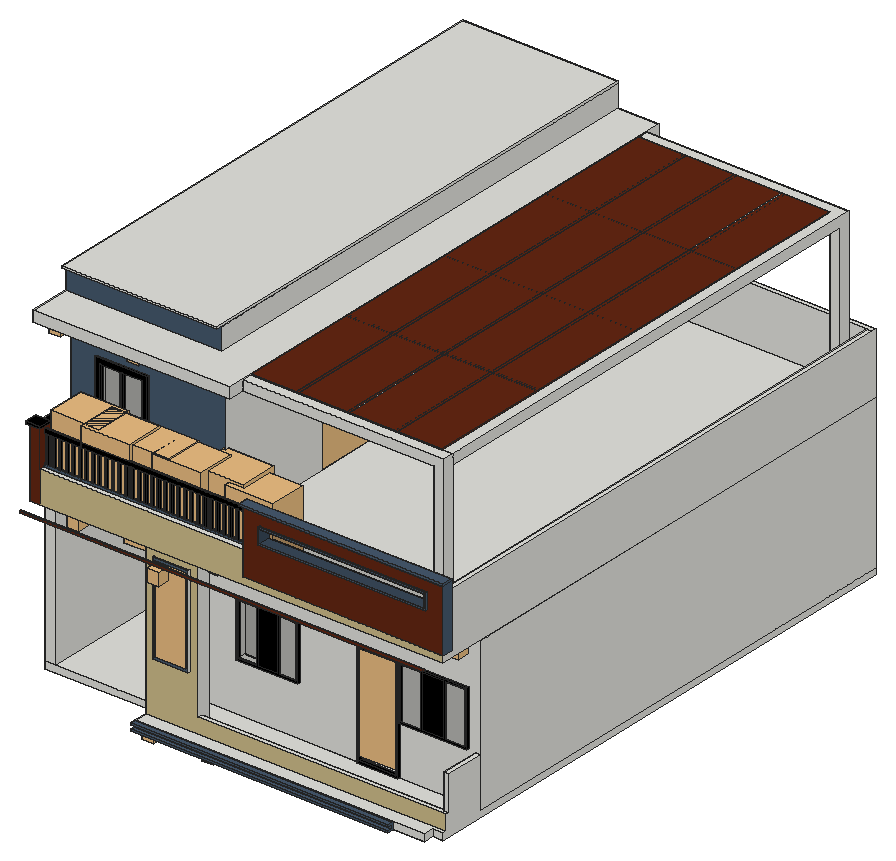
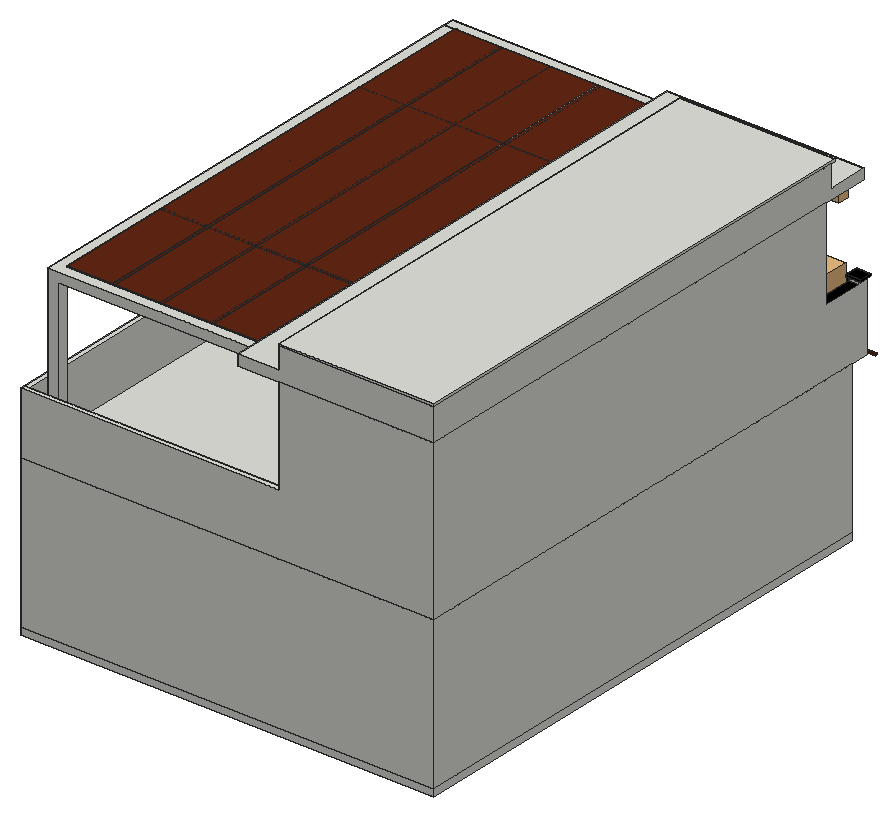
# SketchUp Ruby script. Lengths in inches.
U = 1.inch
M = Sketchup.active_model
def pt(a) = Geom::Point3d.new(a.map { |v| v * U })
def face(e, loops, mat)
  f = e.add_face(loops[0].map { |a| pt(a) })
  loops[1..].each { |l| e.add_face(l.map { |a| pt(a) }).erase! }
  f.material = f.back_material = mat if mat
  f
end
# faces: each face lists its corners as indices into pts; further lists are holes
def faces(e, pts, list, mat = nil) = list.each { |f| face(e, (f[0].is_a?(Array) ? f : [f]).map { |l| l.map { |i| pts[i] } }, mat) }
# xy, xz, yz: faces in a plane at the given z, y or x. An outline is a flat list of corners, or four numbers for a rectangle; further outlines are holes
def ring(l) = l.size == 4 ? [[l[0], l[1]], [l[2], l[1]], [l[2], l[3]], [l[0], l[3]]] : l.each_slice(2).to_a
def flat(e, list, mat, &to3) = list.each { |f| face(e, (f[0].is_a?(Array) ? f : [f]).map { |l| ring(l).map { |u, v| to3.(u, v) } }, mat) }
def xy(e, z, list, mat = nil) = flat(e, list, mat) { |x, y| [x, y, z] }
def xz(e, y, list, mat = nil) = flat(e, list, mat) { |x, z| [x, y, z] }
def yz(e, x, list, mat = nil) = flat(e, list, mat) { |y, z| [x, y, z] }
def lines(e, pts, list) = list.each { |a, b| e.add_line(pt(pts[a]), pt(pts[b])) }
# prism: a flat outline (further loops are holes) pulled along v
def prism(e, loops, v, mat = nil)
  f = face(e, loops, mat); d = Geom::Vector3d.new(v.map { |x| x * U })
  f.pushpull(f.normal.samedirection?(d) ? d.length : -d.length)
end
def box(e, o, s, mat = nil) = prism(e, [[o, [o[0] + s[0], o[1], o[2]], [o[0] + s[0], o[1] + s[1], o[2]], [o[0], o[1] + s[1], o[2]]]], [0, 0, s[2]], mat)
def at(x, y, z, deg = 0) = Geom::Transformation.translation(pt([x, y, z])) * Geom::Transformation.rotation(ORIGIN, Z_AXIS, deg.degrees)
def axes(o, x, y, z) = Geom::Transformation.new([*x, 0, *y, 0, *z, 0, *pt(o).to_a, 1])
def part(name) = M.definitions.add(name)
# library, detail: a bought-in or finely detailed component or shape, given as its bounding box
def library(name, o, s) = part(name).tap { |d| box(d.entities, o, s) }
def detail(e, o, s) = box(e.add_group.entities, o, s)
def put(e, d, t, mat = nil) = e.add_instance(d, t).tap { |i| i.material = mat if mat }
def group(e, t, mat = nil) = e.add_group.tap { |g| g.transformation = t; g.material = mat if mat }.entities
root = M.entities
M.materials.add("GLass").color = [0, 0, 0]
M.materials["GLass"].alpha = 0.1
M.materials.add("Wall Paint Fine Grain 01 Yellow 100cm").color = [207, 190, 139]
M.materials.add("Wall Paint Simple Reflective").color = [70, 89, 109]
M.materials.add("Wood Dark 02 100cm").color = [99, 39, 19]
M.materials.add("metal").color = [0, 0, 0]
c1 = library("Spot Light\#15",[-5.1,-5.1,-11.05],[10.2,10.2,11.05])
c2 = library("Spot Light\#16",[-5.1,-5.1,-11.05],[10.2,10.2,11.05])
c3 = library("Spot Light\#17",[-5.1,-5.1,-11.05],[10.2,10.2,11.05])
c4 = library("Spot Light\#18",[-5.1,-5.1,-11.05],[10.2,10.2,11.05])
c5 = library("Spot Light\#19",[-5.1,-5.1,-11.05],[10.2,10.2,11.05])
c6 = library("Door 01",[-21.26,-2.6,0],[42.52,9.29,84.25])
c7 = library("Group\#119",[0,0,0],[48,96,0.5])
c8 = library("Omni Light\#1",[-12,-12,-12],[24,24,24])
c9 = library("Spot Light\#14",[-5.1,-5.1,-11.05],[10.2,10.2,11.05])
c10 = library("Spot Light\#8",[-5.1,-5.1,-11.05],[10.2,10.2,11.05])
c11 = library("Spot Light\#9",[-5.1,-5.1,-11.05],[10.2,10.2,11.05])
c12 = library("Spot Light\#10",[-5.1,-5.1,-11.05],[10.2,10.2,11.05])
c13 = library("Spot Light\#11",[-5.1,-5.1,-11.05],[10.2,10.2,11.05])
c14 = library("Spot Light\#12",[-5.1,-5.1,-11.05],[10.2,10.2,11.05])
c15 = library("Spot Light\#13",[-5.1,-5.1,-11.05],[10.2,10.2,11.05])
c16 = part("Group\#55")
box(c16.entities,[0,0,-24],[2,1.04,24])
c17 = part("Group\#79")
box(c17.entities,[0,0,-0.2],[41.7,1.97,0.2])
c18 = part("Group\#74")
box(c18.entities,[0,0,-0.2],[39.14,1.97,0.2])
c19 = part("Group\#82")
box(c19.entities,[0,0,-0.2],[39.14,1.97,0.2])
c20 = part("Group\#76")
box(c20.entities,[0,0,-0.2],[1.8,103.4375,0.2])
c21 = part("Group\#81")
box(c21.entities,[0,0,-0.2],[1.8,104.8125,0.2])
c22 = part("Group\#78")
box(c22.entities,[0,0,-0.2],[41.7,1.97,0.2])
c23 = part("Group\#80")
box(c23.entities,[0,0,-0.2],[39.14,1.97,0.2])
c24 = part("Group\#83")
box(c24.entities,[0,0,-0.2],[1.8,101.4375,0.2])
c25 = part("Group\#73")
box(c25.entities,[0,0,0],[2.41,421.5,9])
c26 = library("Monstera deliciosa borsigiana 004",[-20.61,-16.32,0.13],[42.24,32.96,48.74])
c27 = library("Spot Light",[-5.1,-5.1,-11.05],[10.2,10.2,11.05])
c28 = library("Spot Light\#1",[-5.1,-5.1,-11.05],[10.2,10.2,11.05])
c29 = library("Spot Light\#2",[-5.1,-5.1,-11.05],[10.2,10.2,11.05])
c30 = library("Spot Light\#3",[-5.1,-5.1,-11.05],[10.2,10.2,11.05])
c31 = library("Spot Light\#4",[-5.1,-5.1,-11.05],[10.2,10.2,11.05])
c32 = library("Spot Light\#5",[-5.1,-5.1,-11.05],[10.2,10.2,11.05])
c33 = library("Spot Light\#6",[-5.1,-5.1,-11.05],[10.2,10.2,11.05])
c34 = library("Spot Light\#7",[-5.1,-5.1,-11.05],[10.2,10.2,11.05])
put(root,c1,at(303.03,225.95,293.99))
put(root,c2,at(353.32,228.8,293.99))
put(root,c3,at(414.5,235.73,293.99))
put(root,c4,at(475.25,244.97,293.99))
put(root,c5,at(536.13,248.13,293.99))
g1 = group(root,at(314.75,214.125,293.89),"Wall Paint Simple Reflective")
xy(g1,0,[[206.98,-5.03,-17.96,-3.91,-17.93,1.09,207,-0.03]],"Wall Paint Simple Reflective")
xy(g1,6.11,[[206.98,-5.03,207,-0.03,-17.93,1.09,-17.96,-3.91]],"Wall Paint Simple Reflective")
p = [[206.98,-5.03,1.35],[-17.96,-3.91,1.36],[-17.96,-3.91,0],[206.98,-5.03,0],[207,-0.03,0],[207,-0.03,6.11],
  [206.98,-5.03,6.11],[206.98,-5.03,4.77],[207,-1.03,4.77],[207,-1.03,1.35],[-17.9375,0.09,1.36],[-17.9375,0.09,4.79],
  [-17.96,-3.91,4.79],[-17.96,-3.91,6.11],[-17.93,1.09,6.11],[-17.93,1.09,0]]
faces(g1,p,[[0,1,2,3],[4,5,6,7,8,9,0,3],[2,1,10,11,12,13,14,15],[14,5,4,15],[1,0,9,10],[10,9,8,11],[13,12,7,6],[7,12,11,8]],"Wall Paint Simple Reflective")
g2 = group(root,at(197.75,215.125,294))
xy(g2,0,[[99.07,0,99.07,25.84,0,25.84,0,480,360,480,360,9,351,9,351,0]],"Wood Dark 02 100cm")
xy(g2,6,[[99.07,0,351,0,351,9,360,9,360,12,99.07,12],[144.07,16.5,355.5,16.5,355.5,49.79,360,49.79,360,480,0,480,0,25.84,99.07,25.84,99.07,23.84,144.07,23.84]])
xy(g2,19,[[144.07,12,360,12,360,14.84,355.5,14.84,355.5,16.5,144.07,16.5]])
xy(g2,49,[[355.5,14.84,360,49.79]])
xy(g2,52,[[106.07,10,137.07,12]])
xy(g2,54,[[108.07,10,135.07,23.84]])
xy(g2,129,[[108.07,10,135.07,23.84]])
xy(g2,131,[[106.07,10,137.07,12]])
xy(g2,138,[[99.07,12,144.07,23.84]])
xz(g2,0,[[99.07,0,351,6]])
xz(g2,9,[[351,0,360,6]])
xz(g2,10,[[[106.07,52,137.07,131],[108.07,54,135.07,129]]],"Wall Paint Simple Reflective")
xz(g2,12,[[[99.07,6,360,6,360,19,144.07,19,144.07,138,99.07,138],[106.07,52,137.07,131]]],"Wall Paint Fine Grain 01 Yellow 100cm")
xz(g2,14.84,[[355.5,19,360,49]])
xz(g2,16.5,[[144.07,6,355.5,19]])
xz(g2,23.84,[[[99.07,6,144.07,138],[108.07,54,135.07,129]]])
xz(g2,25.84,[[0,0,99.07,6]])
xz(g2,49.79,[[355.5,6,360,49]])
xz(g2,480,[[0,0,360,6]])
yz(g2,0,[[25.84,0,480,6]])
yz(g2,99.07,[[0,0,0,6,12,6,12,138,23.84,138,23.84,6,25.84,6,25.84,0]])
yz(g2,106.07,[[10,52,12,131]])
yz(g2,108.07,[[10,54,23.84,129]])
yz(g2,135.07,[[10,54,23.84,129]])
yz(g2,137.07,[[10,52,12,131]])
yz(g2,144.07,[[16.5,6,23.84,6,23.84,138,12,138,12,19,16.5,19]])
yz(g2,351,[[0,0,9,6]])
yz(g2,355.5,[[16.5,6,16.5,19,14.84,19,14.84,49,49.79,49,49.79,6]])
yz(g2,360,[[9,0,480,0,480,6,49.79,6,49.79,49,14.84,49,14.84,19,12,19,12,6,9,6]])
g3 = group(root,at(196.75,262.23,300))
g4 = group(g3,at(149.5,2.6875,43.44))
xy(g4,0,[[0,-1.79,54.06,0]],"metal")
xy(g4,48.89,[[0,-1.79,54.06,0]],"metal")
xz(g4,-1.79,[[[0,0,54.06,48.89],[1.8,1.63,18.02,47.26],[37.86,1.63,52.26,47.26]]],"metal")
xz(g4,0,[[[0,0,54.06,48.89],[1.8,1.63,52.26,47.26]]],"metal")
yz(g4,0,[[-1.79,0,0,48.89]],"metal")
yz(g4,1.8,[[-1.79,1.63,0,47.26]],"metal")
yz(g4,52.26,[[-1.79,1.63,0,47.26]],"metal")
yz(g4,54.06,[[-1.79,0,0,48.89]],"metal")
g5 = group(g4,at(1.8,-1.79,1.63))
box(g5,[0,0,0],[16.22,0.64,45.63],"GLass")
g6 = group(g4,at(19.82,-1.79,1.63))
box(g6,[0,0,0],[16.22,0.64,45.63],"GLass")
g7 = group(g4,at(37.86,-1.79,1.63))
box(g7,[0,0,0],[14.4,0.64,45.63],"GLass")
g8 = group(g3,at(1,2.6875,0))
xy(g8,0,[[0,-23.95,0,430.21,360,430.21,360,0,289.3,0,289.3,8.07,351,8.07,351,119.92,335.34,119.92,335.34,123.15,351,123.15,351,186.6,226.5,186.6,226.5,279.73,231,279.73,231,189.83,351,189.83,351,315.66,343.72,315.66,343.72,318.89,351,318.89,351,367.29,277.1875,367.29,277.1875,318.89,313.72,318.89,313.72,315.66,226.5,315.66,226.5,318.89,272.6875,318.89,272.6875,383.15,277.1875,383.15,277.1875,370.52,351,370.52,351,422.14,277.1875,422.14,277.1875,414.34,272.6875,414.34,272.6875,422.14,128.6875,422.14,128.6875,318.89,195,318.89,195,315.66,128.6875,315.66,128.6875,239.24,119.6875,239.24,119.6875,422.14,9,422.14,9,-23.95],[117,0,117,8.07,119.6875,8.07,119.6875,143.16,128.6875,143.16,128.6875,97.33,178.5,97.33,178.5,94.11,128.6875,94.11,128.6875,8.07,226.5,8.07,226.5,123.15,299.34,123.15,299.34,119.92,231,119.92,231,8.07,253.3,8.07,253.3,0],[119.6875,186.18,128.6875,239.24]])
xy(g8,43.44,[[148.5,0,202.5,8.07],[289.3,0,349.3,8.07]])
xy(g8,92.33,[[148.5,0,202.5,8.07],[253.3,0,349.3,8.07]])
xy(g8,96,[[178.5,94.11,226.5,97.33],[119.6875,143.16,128.6875,186.18],[226.5,279.73,231,315.66],[195,315.66,226.5,318.89],[313.72,315.66,343.72,318.89],
  [272.6875,383.15,277.1875,414.34]])
xy(g8,97.98,[[299.34,119.92,335.34,123.15]])
xy(g8,132,[[[0,-23.95,9,-23.95,9,422.14,119.6875,422.14,119.6875,8.07,117,8.07,117,0,360,0,360,430.21,0,430.21],[128.6875,97.33,128.6875,315.66,226.5,315.66,226.5,186.6,351,186.6,351,123.15,226.5,123.15,226.5,97.33],[231,189.83,351,315.66],[128.6875,318.89,272.6875,422.14],[231,8.07,351,119.92],[128.6875,8.07,226.5,94.11],[277.1875,370.52,351,422.14],[277.1875,318.89,351,367.29]]])
xz(g8,-23.95,[[0,0,9,132]])
xz(g8,0,[[[117,0,253.3,0,253.3,92.33,349.3,92.33,349.3,43.44,289.3,43.44,289.3,0,360,0,360,132,117,132],[148.5,43.44,202.5,92.33]],[172.5,43.44,202.5,92.33],[289.3,43.44,349.3,92.33]])
xz(g8,8.07,[[117,0,119.6875,132],[[128.6875,0,226.5,132],[148.5,43.44,202.5,92.33]],[231,0,231,132,351,132,351,0,289.3,0,289.3,43.44,349.3,43.44,349.3,92.33,253.3,92.33,253.3,0]])
xz(g8,94.11,[[128.6875,0,178.5,0,178.5,96,226.5,96,226.5,132,128.6875,132]])
xz(g8,97.33,[[128.6875,0,128.6875,132,226.5,132,226.5,96,178.5,96,178.5,0]])
xz(g8,119.92,[[231,0,299.34,0,299.34,97.98,335.34,97.98,335.34,0,351,0,351,132,231,132]])
xz(g8,123.15,[[226.5,0,226.5,132,351,132,351,0,335.34,0,335.34,97.98,299.34,97.98,299.34,0]])
xz(g8,143.16,[[119.6875,0,128.6875,96]])
xz(g8,186.18,[[119.6875,0,128.6875,96]])
xz(g8,186.6,[[226.5,0,351,132]])
xz(g8,189.83,[[231,0,351,132]])
xz(g8,279.73,[[226.5,0,231,96]])
xz(g8,315.66,[[128.6875,0,195,0,195,96,226.5,96,226.5,132,128.6875,132],[226.5,0,313.72,0,313.72,96,343.72,96,343.72,0,351,0,351,132,231,132,231,96,226.5,96]])
xz(g8,318.89,[[128.6875,0,128.6875,132,272.6875,132,272.6875,0,226.5,0,226.5,96,195,96,195,0],[277.1875,0,277.1875,132,351,132,351,0,343.72,0,343.72,96,313.72,96,313.72,0]])
xz(g8,367.29,[[277.1875,0,351,132]])
xz(g8,370.52,[[277.1875,0,351,132]])
xz(g8,383.15,[[272.6875,0,277.1875,96]])
xz(g8,414.34,[[272.6875,0,277.1875,96]])
xz(g8,422.14,[[9,0,119.6875,132],[128.6875,0,272.6875,132],[277.1875,0,351,132]])
xz(g8,430.21,[[0,0,360,132]])
yz(g8,0,[[-23.95,0,430.21,132]])
yz(g8,9,[[-23.95,0,422.14,132]])
yz(g8,117,[[0,0,8.07,132]])
yz(g8,119.6875,[[8.07,0,8.07,132,422.14,132,422.14,0,186.18,0,186.18,96,143.16,96,143.16,0]])
yz(g8,128.6875,[[8.07,0,94.11,132],[97.33,0,143.16,0,143.16,96,186.18,96,186.18,0,315.66,0,315.66,132,97.33,132],[318.89,0,422.14,132]])
yz(g8,178.5,[[94.11,0,97.33,96]])
yz(g8,195,[[315.66,0,318.89,96]])
yz(g8,202.5,[[0,43.44,8.07,92.33]])
yz(g8,226.5,[[8.07,0,8.07,132,94.11,132,94.11,96,97.33,96,97.33,132,123.15,132,123.15,0],[186.6,0,186.6,132,315.66,132,315.66,96,279.73,96,279.73,0],[315.66,0,318.89,96]])
yz(g8,231,[[8.07,0,119.92,132],[189.83,0,279.73,0,279.73,96,315.66,96,315.66,132,189.83,132]])
yz(g8,253.3,[[0,0,8.07,92.33]])
yz(g8,272.6875,[[318.89,0,318.89,132,422.14,132,422.14,0,414.34,0,414.34,96,383.15,96,383.15,0]])
yz(g8,277.1875,[[318.89,0,367.29,132],[370.52,0,383.15,0,383.15,96,414.34,96,414.34,0,422.14,0,422.14,132,370.52,132]])
yz(g8,289.3,[[0,0,8.07,43.44]])
yz(g8,299.34,[[119.92,0,123.15,97.98]])
yz(g8,313.72,[[315.66,0,318.89,96]])
yz(g8,335.34,[[119.92,0,123.15,97.98]])
yz(g8,343.72,[[315.66,0,318.89,96]])
yz(g8,349.3,[[0,43.44,8.07,92.33]])
yz(g8,351,[[8.07,0,119.92,132],[123.15,0,186.6,132],[189.83,0,315.66,132],[318.89,0,367.29,132],[370.52,0,422.14,132]])
yz(g8,360,[[0,0,430.21,132]])
p = [[313.72,315.66,0],[343.72,315.66,0],[226.5,279.73,0],[226.5,315.66,0],[272.6875,414.34,0],[272.6875,383.15,0],
  [195,315.66,0],[119.6875,186.18,0],[119.6875,143.16,0],[335.34,123.15,0],[299.34,123.15,0]]
lines(g8,p,[[0,1],[2,3],[4,5],[3,6],[7,8],[9,10]])
g9 = group(g8,at(253.3,0,0))
prism(g9,[[[0,1.79,0],[0,1.79,92.33],[36,1.79,92.33],[36,1.79,0]],[[34,1.79,2],[34,1.79,90.33],[2,1.79,90.33],[2,1.79,2]]],[0,-3.59,0],"metal")
g10 = group(g8,at(313.72,315.66,0))
prism(g10,[[[30,0,0],[30,0,96],[0,0,96],[0,0,0]],[[28,0,2],[2,0,2],[2,0,94],[28,0,94]]],[0,2,0])
g11 = group(g8,at(226.5,279.73,0))
prism(g11,[[[0,35.9375,0],[0,0,0],[0,0,96],[0,35.9375,96]],[[0,33.9375,94],[0,2,94],[0,2,2],[0,33.9375,2]]],[2,0,0])
g12 = group(g8,at(272.6875,383.15,0))
prism(g12,[[[0,0,0],[0,0,96],[0,31.2,96],[0,31.2,0]],[[0,2,94],[0,2,2],[0,29.2,2],[0,29.2,94]]],[2,0,0])
g13 = group(g8,at(195,315.66,0))
prism(g13,[[[0,0,96],[0,0,0],[31.5,0,0],[31.5,0,96]],[[2,0,2],[2,0,94],[29.5,0,94],[29.5,0,2]]],[0,2,0])
g14 = group(g8,at(119.6875,143.16,0))
prism(g14,[[[0,0,0],[0,0,96],[0,43.02,96],[0,43.02,0]],[[0,2,94],[0,2,2],[0,41.02,2],[0,41.02,94]]],[2,0,0])
g15 = group(g8,at(299.34,123.15,0))
prism(g15,[[[0,0,0],[0,0,97.98],[36,0,97.98],[36,0,0]],[[2,0,95.98],[2,0,2],[34,0,2],[34,0,95.98]]],[0,-2,0])
g16 = group(g3,at(290.3,2.6875,43.44))
xy(g16,0,[[0,-1.79,60,1.79]],"metal")
xy(g16,48.89,[[0,-1.79,60,1.79]],"metal")
xz(g16,-1.79,[[[0,0,60,48.89],[2,1.63,20,47.26],[42.01,1.63,58,47.26]]],"metal")
xz(g16,1.79,[[[0,0,60,48.89],[2,1.63,58,47.26]]],"metal")
yz(g16,0,[[-1.79,0,1.79,48.89]],"metal")
yz(g16,2,[[-1.79,1.63,1.79,47.26]],"metal")
yz(g16,58,[[-1.79,1.63,1.79,47.26]],"metal")
yz(g16,60,[[-1.79,0,1.79,48.89]],"metal")
g17 = group(g16,at(2,-1.79,1.63))
box(g17,[0,0,0],[18,0.64,45.63],"GLass")
g18 = group(g16,at(22,-1.79,1.63))
box(g18,[0,0,0],[18,0.64,45.63],"GLass")
g19 = group(g16,at(42.01,-1.79,1.63))
box(g19,[0,0,0],[15.99,0.64,45.63],"GLass")
put(root,c6,axes([469.04,264.13,306.08],[0.75321,0,0],[0,-0.15,0],[0,0,1]))
put(root,c7,axes([305.82,225.625,348.12],[0.5625,0,0],[0,0,0.78],[0,-1,0]))
put(root,c8,at(241.81,298.61,395.6875))
put(root,c9,at(317.18,213.78,426.99))
put(root,c10,at(345.41,243.44,431.99))
put(root,c11,at(401.08,246.11,431.99))
put(root,c12,at(461.41,248.79,431.99))
put(root,c13,at(508.5,251.9375,431.99))
put(root,c14,at(545.66,254.75,431.99))
put(root,c15,at(233.05,232.41,431.99))
g20 = group(root,at(197.75,214.125,427))
prism(g20,[[[0,1,0],[351,0,0],[351,-1,0],[0,0,0]]],[0,0,2],"Wood Dark 02 100cm")
g21 = group(root,at(197.75,215.125,432))
xy(g21,0,[[0,9,360,480]],"Wood Dark 02 100cm")
xy(g21,6,[[186,9,355.5,9,355.5,475.5,135,475.5,135,218.43,126,218.43,126,471,9,471,9,63,126,63,126,159.1,135,159.1,135,54,9,54,9,18,186,18],[355.5,9,360,18]])
xy(g21,28.5,[[9,9,186,18]])
xy(g21,40.5,[[22.5,54,67.5,63]])
xy(g21,54,[[355.5,18,360,475.5],[126,304.11,135,377.17],[135,475.5,360,480]])
xy(g21,58.5,[[0,18,9,54]],"metal")
xy(g21,60.75,[[0,9,9,18]])
xy(g21,102,[[22.5,54,67.5,63],[126,159.1,135,218.43],[126,304.11,135,377.17]])
xy(g21,138,[[[0,54,135,480],[9,63,126,471]]])
xz(g21,9,[[9,0,360,0,360,6,186,6,186,28.5,9,28.5]],"Wall Paint Fine Grain 01 Yellow 100cm")
xz(g21,9,[[0,0,9,60.75]],"Wood Dark 02 100cm")
xz(g21,18,[[9,6,186,28.5],[355.5,6,360,54],[0,58.5,9,60.75]])
xz(g21,54,[[[9,6,135,6,135,138,0,138,0,58.5,9,58.5],[22.5,40.5,67.5,102]]],"Wall Paint Simple Reflective")
xz(g21,63,[[[9,6,126,138],[22.5,40.5,67.5,102]]])
xz(g21,159.1,[[126,6,135,102]])
xz(g21,218.43,[[126,6,135,102]])
xz(g21,304.11,[[126,54,135,102]])
xz(g21,377.17,[[126,54,135,102]])
xz(g21,471,[[9,6,126,138]])
xz(g21,475.5,[[135,6,355.5,54]])
xz(g21,480,[[0,0,0,138,135,138,135,54,360,54,360,0]])
yz(g21,0,[[9,0,9,60.75,18,60.75,18,58.5,54,58.5,54,138,480,138,480,0]])
yz(g21,9,[[63,6,471,138]])
yz(g21,9,[[18,6,54,6,54,58.5,18,58.5,18,60.75,9,60.75,9,28.5,18,28.5]],"Wood Dark 02 100cm")
yz(g21,22.5,[[54,40.5,63,102]])
yz(g21,67.5,[[54,40.5,63,102]])
yz(g21,126,[[[63,6,63,138,471,138,471,6,218.43,6,218.43,102,159.1,102,159.1,6],[304.11,54,377.17,102]]])
yz(g21,135,[[[54,6,159.1,6,159.1,102,218.43,102,218.43,6,475.5,6,475.5,54,480,54,480,138,54,138],[304.11,54,377.17,102]]])
yz(g21,186,[[9,6,18,28.5]])
yz(g21,355.5,[[18,6,475.5,54]])
yz(g21,360,[[9,0,480,0,480,54,18,54,18,6,9,6]])
g22 = group(g21,at(9,12.98,28.5),"Wall Paint Simple Reflective")
box(g22,[0,0,0],[177,1.04,2],"Wall Paint Simple Reflective")
g23 = group(g21,at(9,12.98,54.5),"metal")
box(g23,[0,0,0],[177,1.04,4])
g24 = group(g21,at(0,9,60.75),"metal")
box(g24,[-2,-2,0],[13,11,2])
put(g21,c16,at(10.98,12.98,54.5),"metal")
put(g21,c16,at(16.68,12.98,54.5),"metal")
put(g21,c16,at(22.38,12.98,54.5),"metal")
put(g21,c16,at(28.09,12.98,54.5),"metal")
put(g21,c16,at(33.79,12.98,54.5),"metal")
put(g21,c16,at(39.49,12.98,54.5),"metal")
put(g21,c16,at(45.19,12.98,54.5),"metal")
put(g21,c16,at(50.89,12.98,54.5),"metal")
put(g21,c16,at(56.6,12.98,54.5),"metal")
put(g21,c16,at(62.3,12.98,54.5),"metal")
put(g21,c16,at(68,12.98,54.5),"metal")
put(g21,c16,at(73.7,12.98,54.5),"metal")
put(g21,c16,at(79.4,12.98,54.5),"metal")
put(g21,c16,at(85.11,12.98,54.5),"metal")
put(g21,c16,at(90.81,12.98,54.5),"metal")
put(g21,c16,at(96.51,12.98,54.5),"metal")
put(g21,c16,at(102.21,12.98,54.5),"metal")
put(g21,c16,at(107.91,12.98,54.5),"metal")
put(g21,c16,at(113.62,12.98,54.5),"metal")
put(g21,c16,at(119.32,12.98,54.5),"metal")
put(g21,c16,at(125.02,12.98,54.5),"metal")
put(g21,c16,at(130.72,12.98,54.5),"metal")
put(g21,c16,at(136.42,12.98,54.5),"metal")
put(g21,c16,at(142.13,12.98,54.5),"metal")
put(g21,c16,at(147.83,12.98,54.5),"metal")
put(g21,c16,at(153.53,12.98,54.5),"metal")
put(g21,c16,at(159.23,12.98,54.5),"metal")
put(g21,c16,at(164.94,12.98,54.5),"metal")
put(g21,c16,at(170.64,12.98,54.5),"metal")
put(g21,c16,at(176.34,12.98,54.5),"metal")
put(g21,c16,at(182.04,12.98,54.5),"metal")
g25 = group(g21,at(186,9,6))
xy(g25,0,[[0,0,174,9]],"Wall Paint Simple Reflective")
xy(g25,31,[[14,-2,160.09,0]],"Wall Paint Simple Reflective")
xy(g25,32,[[15,-2,159,9]],"Wall Paint Simple Reflective")
xy(g25,44,[[15,-2,159,9]],"Wall Paint Simple Reflective")
xy(g25,45,[[14,-2,160.09,0]],"Wall Paint Simple Reflective")
xy(g25,54,[[0,0,174,9]],"Wall Paint Simple Reflective")
xz(g25,-2,[[[14,31,160.09,45],[15,32,159,44]]],"Wall Paint Simple Reflective")
xz(g25,0,[[[0,0,174,54],[14,31,160.09,45]]],"Wood Dark 02 100cm")
xz(g25,9,[[[0,0,174,54],[15,32,159,44]]],"Wall Paint Simple Reflective")
yz(g25,0,[[0,0,9,54]],"Wall Paint Simple Reflective")
yz(g25,14,[[-2,31,0,45]],"Wall Paint Simple Reflective")
yz(g25,15,[[-2,32,9,44]],"Wall Paint Simple Reflective")
yz(g25,159,[[-2,32,9,44]],"Wall Paint Simple Reflective")
yz(g25,160.09,[[-2,31,0,45]],"Wall Paint Simple Reflective")
yz(g25,174,[[0,0,9,54]],"Wall Paint Simple Reflective")
g26 = group(g21,at(186,9,60),"Wall Paint Simple Reflective")
box(g26,[-3.96,0,0],[177.96,9,2],"Wall Paint Simple Reflective")
g27 = group(g21,at(22.5,54,40.5))
prism(g27,[[[45,-2,0],[45,-2,61.5],[0,-2,61.5],[0,-2,0]],[[4.5,-2,57],[21.26,-2,57],[21.26,-2,4.5],[4.5,-2,4.5]],[[23.74,-2,4.5],[23.74,-2,57],[40.5,-2,57],[40.5,-2,4.5]]],[0,3,0],"metal")
g28 = group(g21,at(135,159.1,6),"metal")
prism(g28,[[[0,59.33,0],[0,59.33,96],[0,0,96],[0,0,0]],[[0,57.33,2],[0,2,2],[0,2,94],[0,57.33,94]]],[-2.5,0,0])
g29 = group(g21,at(135,304.11,54))
prism(g29,[[[1.5,73.06,0],[1.5,73.06,48],[1.5,0,48],[1.5,0,0]],[[1.5,2,2],[1.5,2,46],[1.5,71.06,46],[1.5,71.06,2]]],[-3,0,0],"metal")
g30 = group(g29,at(-0.375,2,2))
box(g30,[-0.31,0,0],[0.31,34.53,44],"GLass")
g31 = group(g29,at(-0.06,36.53,2))
box(g31,[-0.31,0,0],[0.31,34.53,44],"GLass")
g32 = group(root,at(366.8125,242.125,438))
put(g32,c17,at(41.55,191.53,132.15))
put(g32,c17,at(41.55,186.4,132.14))
put(g32,c18,at(127.36,114.625,132))
put(g32,c17,at(41.55,119.75,132.01))
put(g32,c17,at(41.55,212.04,132.19))
put(g32,c17,at(41.55,135.13,132.04))
put(g32,c17,at(41.55,124.88,132.02))
put(g32,c17,at(41.55,130.01,132.03))
put(g32,c17,at(41.55,165.89,132.1))
put(g32,c19,at(85.79,100.32,132.18))
put(g32,c20,at(54.85,9,132.07))
put(g32,c19,at(85.74,64.81,132.11))
put(g32,c19,at(85.8,105.4,132.19))
put(g32,c19,at(0,34.37,132))
put(g32,c21,at(0,114.625,132.2))
put(g32,c19,at(0,59.73,132))
put(g32,c19,at(85.75,69.88,132.12))
put(g32,c19,at(0,74.95,132))
put(g32,c19,at(0,110.47,132))
put(g32,c19,at(0,44.51,132))
put(g32,c20,at(61.5,9,132.1))
put(g32,c19,at(85.6875,29.29,132.04))
put(g32,c19,at(85.72,49.59,132.08))
put(g32,c19,at(0,100.32,132))
put(g32,c19,at(0,85.1,132))
put(g32,c19,at(0,95.25,132))
put(g32,c19,at(85.76,80.03,132.14))
put(g32,c19,at(85.77,85.1,132.15))
put(g32,c19,at(0,105.4,132))
put(g32,c19,at(85.67,19.15,132.02))
put(g32,c19,at(0,9,132))
put(g32,c19,at(0,14.07,132))
put(g32,c19,at(0,24.22,132))
put(g32,c19,at(0,19.15,132))
put(g32,c20,at(48.2,9,132.03))
put(g32,c20,at(68.15,9,132.13))
put(g32,c19,at(85.7,34.37,132.05))
put(g32,c20,at(81.45,9,132.2))
put(g32,c19,at(85.73,59.73,132.1))
put(g32,c19,at(85.78,90.17,132.16))
put(g32,c19,at(85.7,39.44,132.06))
put(g32,c19,at(0,69.88,132))
put(g32,c19,at(85.66,9,132))
put(g32,c19,at(85.79,95.25,132.17))
put(g32,c20,at(127.36,9,132.2))
put(g32,c19,at(0,90.17,132))
put(g32,c19,at(0,49.59,132))
put(g32,c20,at(74.8,9,132.17))
put(g32,c17,at(41.55,201.78,132.17))
put(g32,c19,at(85.73,54.66,132.09))
put(g32,c19,at(85.76,74.95,132.13))
put(g32,c19,at(0,54.66,132))
g33 = group(g32,at(0,64.81,132))
box(g33,[0,0,-0.2],[39.14,1.97,0.2])
put(g32,c19,at(0,80.03,132))
put(g32,c19,at(0,39.44,132))
put(g32,c19,at(85.67,14.07,132.01))
put(g32,c19,at(85.68,24.22,132.03))
put(g32,c19,at(85.71,44.51,132.07))
put(g32,c19,at(0,29.29,132))
put(g32,c19,at(85.81,110.47,132.2))
put(g32,c20,at(139.81,9,132.2))
put(g32,c20,at(133.58,9,132.2))
put(g32,c17,at(41.55,171.02,132.11))
put(g32,c22,axes([127.36,368.85,132.2],[0.93866,0,0],[0,1,0],[0,0,1]))
put(g32,c22,axes([127.36,363.875,132.2],[0.93866,0,0],[0,1,0],[0,0,1]))
put(g32,c22,axes([127.36,339.01,132.2],[0.93866,0,0],[0,1,0],[0,0,1]))
put(g32,c22,axes([127.36,413.61,132.2],[0.93866,0,0],[0,1,0],[0,0,1]))
put(g32,c22,axes([127.36,348.96,132.2],[0.93866,0,0],[0,1,0],[0,0,1]))
put(g32,c22,axes([127.36,343.98,132.2],[0.93866,0,0],[0,1,0],[0,0,1]))
put(g32,c22,axes([127.36,353.93,132.2],[0.93866,0,0],[0,1,0],[0,0,1]))
put(g32,c22,axes([127.36,358.9,132.2],[0.93866,0,0],[0,1,0],[0,0,1]))
put(g32,c22,at(41.55,348.95,132.2))
put(g32,c22,at(41.55,343.98,132.2))
put(g32,c22,at(41.55,358.89,132.2))
put(g32,c22,at(41.55,353.92,132.2))
put(g32,c22,at(41.55,339.01,132.2))
put(g32,c22,at(41.55,368.84,132.2))
put(g32,c22,at(41.55,363.87,132.2))
put(g32,c21,at(127.36,222,132.2))
put(g32,c22,axes([127.36,378.8,132.2],[0.93866,0,0],[0,1,0],[0,0,1]))
put(g32,c22,at(41.55,334.03,132.2))
put(g32,c22,at(41.55,373.81,132.2))
put(g32,c23,at(85.66,273.27,132.1))
put(g32,c23,at(85.66,293.9,132.14))
put(g32,c23,at(85.66,309.37,132.17))
put(g32,c23,at(85.66,283.58,132.12))
put(g32,c23,at(85.66,314.53,132.18))
put(g32,c23,at(85.66,278.42,132.11))
put(g32,c23,at(85.66,268.11,132.09))
put(g32,c23,at(85.66,304.21,132.16))
put(g32,c23,at(85.66,324.84,132.2))
put(g32,c23,at(85.66,319.6875,132.19))
put(g32,c23,at(85.66,299.05,132.15))
put(g32,c23,at(85.66,288.74,132.13))
put(g32,c20,at(152.25,9,132.2))
put(g32,c21,at(18.66,114.625,132.2))
put(g32,c20,at(164.7,9,132.2))
put(g32,c20,at(146.03,9,132.2))
put(g32,c21,at(31.09,114.625,132.2))
put(g32,c21,at(24.875,114.625,132.2))
put(g32,c21,at(37.3125,114.625,132.2))
put(g32,c21,at(12.4375,114.625,132.2))
put(g32,c21,at(6.22,114.625,132.2))
put(g32,c17,at(41.55,114.625,132))
put(g32,c20,at(158.48,9,132.2))
put(g32,c18,at(127.36,171.14,132))
put(g32,c18,at(127.36,186.55,132))
put(g32,c18,at(127.36,196.82,132))
put(g32,c18,at(127.36,201.96,132))
put(g32,c18,at(127.36,217.375,132))
put(g32,c21,at(91.88,114.625,132.2))
put(g32,c21,at(98.13,114.625,132.2))
put(g32,c21,at(110.64,114.625,132.2))
put(g32,c21,at(116.9,114.625,132.2))
put(g32,c18,at(127.36,155.72,132))
put(g32,c21,at(123.15,114.625,132.2))
put(g32,c18,at(127.36,140.3125,132))
put(g32,c18,at(127.36,145.45,132))
put(g32,c18,at(127.36,207.1,132))
put(g32,c18,at(127.36,119.76,132))
put(g32,c18,at(127.36,135.17,132))
put(g32,c18,at(127.36,166,132))
put(g32,c18,at(127.36,130.04,132))
put(g32,c18,at(127.36,191.6875,132))
put(g32,c23,at(0,221.6875,132))
put(g32,c18,at(127.36,212.24,132))
put(g32,c18,at(127.36,124.9,132))
put(g32,c21,at(85.625,114.625,132.2))
put(g32,c18,at(127.36,150.59,132))
put(g32,c21,at(104.39,114.625,132.2))
put(g32,c18,at(127.36,160.86,132))
put(g32,c18,at(127.36,176.27,132))
put(g32,c18,at(127.36,181.41,132))
put(g32,c24,at(6.22,329.0625,132))
put(g32,c24,at(24.9,329.0625,132))
g34 = group(g32,at(18.67,329.0625,132))
box(g34,[0,0,-0.2],[1.8,101.4375,0.2])
put(g32,c24,at(12.45,329.0625,132))
put(g32,c24,at(37.35,329.0625,132))
put(g32,c24,at(85.66,329.0625,132))
put(g32,c24,at(98.16,329.0625,132.07))
put(g32,c24,at(123.15,329.0625,132.2))
put(g32,c24,at(91.91,329.0625,132.03))
put(g32,c24,at(104.41,329.0625,132.1))
put(g32,c24,at(110.65,329.0625,132.13))
put(g32,c24,at(116.9,329.0625,132.17))
put(g32,c21,at(81.45,222,132.2))
put(g32,c21,at(48.2,222,132.2))
put(g32,c21,at(68.15,222,132.2))
put(g32,c22,axes([127.36,423.56,132.2],[0.93866,0,0],[0,1,0],[0,0,1]))
put(g32,c21,at(74.8,222,132.2))
put(g32,c21,at(61.5,222,132.2))
put(g32,c22,axes([127.36,428.53,132.2],[0.93866,0,0],[0,1,0],[0,0,1]))
put(g32,c21,at(41.55,222,132.2))
put(g32,c21,at(54.85,222,132.2))
put(g32,c22,axes([127.36,418.58,132.2],[0.93866,0,0],[0,1,0],[0,0,1]))
put(g32,c22,at(41.55,398.67,132.2))
put(g32,c22,at(41.55,413.58,132.2))
put(g32,c22,at(41.55,378.78,132.2))
put(g32,c22,at(41.55,428.5,132.2))
put(g32,c22,axes([127.36,334.04,132.2],[0.93866,0,0],[0,1,0],[0,0,1]))
put(g32,c22,at(41.55,393.7,132.2))
put(g32,c22,axes([127.36,373.82,132.2],[0.93866,0,0],[0,1,0],[0,0,1]))
put(g32,c22,at(41.55,418.56,132.2))
put(g32,c22,axes([127.36,329.0625,132.2],[0.93866,0,0],[0,1,0],[0,0,1]))
put(g32,c22,at(41.55,403.64,132.2))
put(g32,c22,at(41.55,408.61,132.2))
put(g32,c22,at(41.55,383.75,132.2))
put(g32,c22,at(41.55,388.72,132.2))
put(g32,c22,at(41.55,423.53,132.2))
put(g32,c23,at(85.66,257.79,132.07))
put(g32,c23,at(0,268.11,132))
put(g32,c23,at(0,273.27,132))
put(g32,c23,at(0,252.63,132))
put(g32,c23,at(0,262.95,132))
put(g32,c23,at(0,257.79,132))
put(g32,c23,at(0,283.58,132))
put(g32,c23,at(0,278.42,132))
put(g32,c22,axes([127.36,408.64,132.2],[0.93866,0,0],[0,1,0],[0,0,1]))
put(g32,c22,axes([127.36,403.66,132.2],[0.93866,0,0],[0,1,0],[0,0,1]))
put(g32,c22,axes([127.36,398.69,132.2],[0.93866,0,0],[0,1,0],[0,0,1]))
put(g32,c22,axes([127.36,388.74,132.2],[0.93866,0,0],[0,1,0],[0,0,1]))
put(g32,c22,axes([127.36,393.72,132.2],[0.93866,0,0],[0,1,0],[0,0,1]))
put(g32,c22,axes([127.36,383.77,132.2],[0.93866,0,0],[0,1,0],[0,0,1]))
put(g32,c21,at(133.58,222,132.2))
put(g32,c24,at(31.12,329.0625,132))
put(g32,c23,at(0,247.48,132))
put(g32,c23,at(0,237.16,132))
put(g32,c23,at(0,242.32,132))
put(g32,c23,at(0,226.85,132))
put(g32,c23,at(0,288.74,132))
put(g32,c23,at(0,232,132))
put(g32,c23,at(85.66,252.63,132.06))
put(g32,c21,at(158.48,222,132.2))
put(g32,c21,at(164.7,222,132.2))
put(g32,c21,at(139.81,222,132.2))
put(g32,c24,at(0,329.0625,132))
put(g32,c21,at(146.03,222,132.2))
put(g32,c21,at(152.25,222,132.2))
put(g32,c23,at(0,324.84,132))
put(g32,c23,at(85.66,221.6875,132))
put(g32,c23,at(0,304.21,132))
put(g32,c23,at(85.66,232,132.02))
put(g32,c23,at(0,309.37,132))
put(g32,c23,at(85.66,226.85,132.01))
put(g32,c23,at(85.66,262.95,132.08))
put(g32,c23,at(85.66,237.16,132.03))
put(g32,c23,at(0,293.9,132))
put(g32,c23,at(0,299.05,132))
put(g32,c22,at(41.55,329.0625,132.2))
put(g32,c23,at(85.66,242.32,132.04))
put(g32,c23,at(85.66,247.48,132.05))
put(g32,c23,at(0,314.53,132))
put(g32,c23,at(0,319.6875,132))
put(g32,c17,at(41.55,217.16,132.2))
put(g32,c17,at(41.55,176.15,132.12))
put(g32,c17,at(41.55,206.91,132.18))
put(g32,c17,at(41.55,181.27,132.13))
put(g32,c17,at(41.55,155.64,132.08))
put(g32,c17,at(41.55,160.77,132.09))
put(g32,c17,at(41.55,145.39,132.06))
g35 = group(g32,at(1.9375,0,0))
g36 = group(g35,at(166.5,0,0))
xy(g36,0,[[0,0,9,9]])
xy(g36,141,[[-166.5,0,9,9]])
xz(g36,0,[[0,0,9,0,9,141,-166.5,141,-166.5,132,0,132]])
xz(g36,9,[[0,0,0,132,-166.5,132,-166.5,141,9,141,9,0]])
yz(g36,-166.5,[[0,132,9,141]])
yz(g36,0,[[0,0,9,132]])
yz(g36,9,[[0,0,9,141]])
g37 = group(g36,at(-166.5,0,132))
xy(g37,0,[[0,0,166.5,9]])
g38 = group(g36,at(-166.5,107.625,132))
box(g38,[0,4.8125,0],[166.5,2.1875,9])
g39 = group(g36,at(-166.5,215.25,132))
box(g39,[0,4.1875,0],[166.5,2.25,9])
g40 = group(g36,at(-166.5,322.875,132))
box(g40,[0,3.9375,0],[166.5,2.25,9])
g41 = group(g35,at(166.5,430.5,0))
xy(g41,0,[[0,0,9,9]])
xy(g41,132,[[0,-421.5,9,0],[-166.5,0,0,9]])
xy(g41,141,[[0,-421.5,9,-421.5,9,9,-166.5,9,-166.5,0,0,0]])
xz(g41,-421.5,[[0,132,9,141]])
xz(g41,0,[[0,0,9,132],[-166.5,132,0,141]])
xz(g41,9,[[0,0,0,132,-166.5,132,-166.5,141,9,141,9,0]])
yz(g41,-166.5,[[0,132,9,141]])
yz(g41,0,[[0,0,9,132],[-421.5,132,0,141]])
yz(g41,9,[[0,0,9,0,9,141,-421.5,141,-421.5,132,0,132]])
g42 = group(g35,at(0,9,141),"Wood Dark 02 100cm")
box(g42,[0,0,0],[166.5,421.5,0.31],"Wood Dark 02 100cm")
put(g35,c25,at(39.14,9,132))
put(g35,c25,at(83.25,9,132))
put(g35,c25,at(124.95,9,132))
put(g32,c17,at(41.55,196.66,132.16))
put(g32,c17,at(41.55,140.26,132.05))
put(g32,c17,at(41.55,150.51,132.07))
put(root,c26,axes([319.8,247.2,437.96],[1,0,0],[0,1,0],[0,0,1.29924]))
put(root,c26,axes([259.48,245.11,437.96],[1,0,0],[0,1,0],[0,0,1.33606]))
put(root,c26,axes([229.97,248.63,437.96],[1,0,0],[0,1,0],[0,0,1.33606]))
put(root,c26,axes([351.3,254.71,437.96],[1,0,0],[0,1,0],[0,0,1.27384]))
put(root,c26,axes([291.1,247.89,437.96],[1,0,0],[0,1,0],[0,0,1.30994]))
put(root,c26,axes([380.76,249.34,437.97],[1,0,0],[0,1,0],[0,0,1.2222]))
put(root,c6,axes([333.13,398.07,440],[0,1.1904,0],[0.14699,0,0],[0,0,1.10449]))
g43 = group(root,at(398.75,222.125,470))
box(g43,[0,0,0],[144,0.31,12],"GLass")
g44 = group(root,at(224.75,268.625,477))
box(g44,[0,0,0],[16.76,0.31,52.5],"GLass")
g45 = group(root,at(243.99,269.0625,477))
box(g45,[0,0,0],[16.76,0.31,52.5],"GLass")
put(root,c27,at(207.87,243.73,569.99))
put(root,c28,at(274.64,245.72,569.99))
put(root,c29,at(346.05,252.76,569.99))
put(root,c30,at(343.87,313.51,569.99))
put(root,c31,at(347.57,391.8,569.99))
put(root,c32,at(344.79,478.74,569.99))
put(root,c33,at(346.42,571.49,569.99))
put(root,c34,at(346.9,674.29,569.99))
g46 = group(root,at(197.75,269.125,570))
xy(g46,0,[[0,-41.02,171,426]],"Wood Dark 02 100cm")
xy(g46,9,[[0,-41.02,171,-41.02,171,426,135,426,135,-5.02,0,-5.02],[3.55,-0.52,131.45,421.5]])
xy(g46,28,[[0,-5.02,135,-5.02,135,426,0,426,0,421.5,131.45,421.5,131.45,-0.52,3.55,-0.52,3.55,421.5,0,421.5]])
xz(g46,-41.02,[[0,0,171,9]])
xz(g46,-5.02,[[0,9,135,28]],"Wall Paint Simple Reflective")
xz(g46,-0.52,[[3.55,9,131.45,28]])
xz(g46,421.5,[[3.55,9,131.45,28]])
xz(g46,426,[[0,0,0,28,135,28,135,9,171,9,171,0]])
yz(g46,0,[[-41.02,0,-41.02,9,-5.02,9,-5.02,28,426,28,426,0]])
yz(g46,3.55,[[-0.52,9,421.5,28]])
yz(g46,131.45,[[-0.52,9,421.5,28]])
yz(g46,135,[[-5.02,9,426,28]])
yz(g46,171,[[-41.02,0,426,9]])
g47 = group(root,at(201.3,268.6,598))
box(g47,[-3.55,-9.1875,0],[135,435.71,2])
